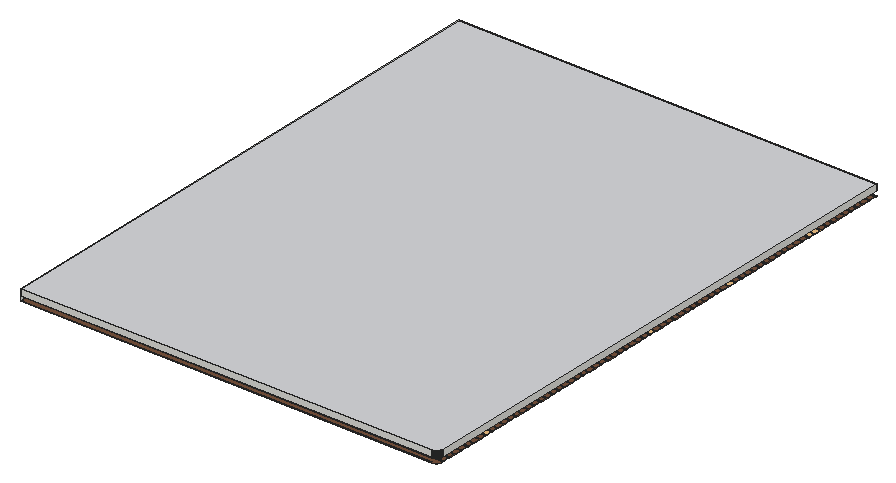
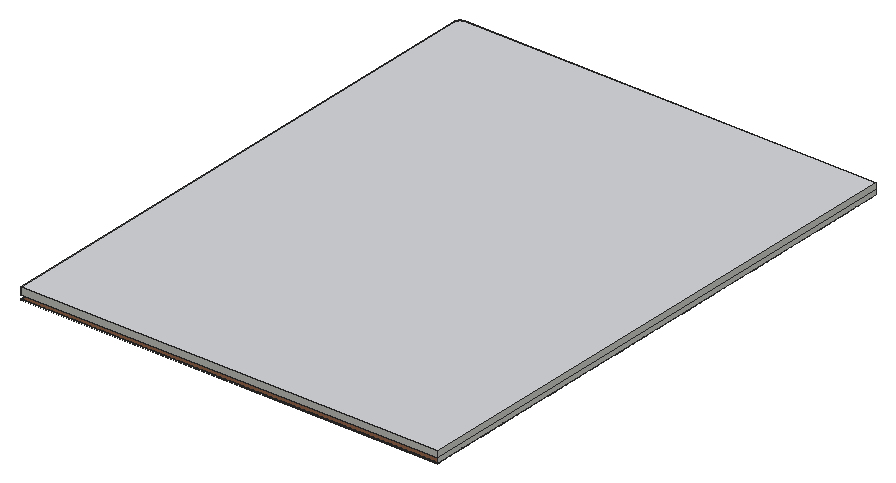
# SketchUp Ruby script. Lengths in inches.
U = 1.inch
M = Sketchup.active_model
def pt(a) = Geom::Point3d.new(a.map { |v| v * U })
def face(e, loops, mat)
  f = e.add_face(loops[0].map { |a| pt(a) })
  loops[1..].each { |l| e.add_face(l.map { |a| pt(a) }).erase! }
  f.material = f.back_material = mat if mat
  f
end
# faces: each face lists its corners as indices into pts; further lists are holes
def faces(e, pts, list, mat = nil) = list.each { |f| face(e, (f[0].is_a?(Array) ? f : [f]).map { |l| l.map { |i| pts[i] } }, mat) }
# xy, xz, yz: faces in a plane at the given z, y or x. An outline is a flat list of corners, or four numbers for a rectangle; further outlines are holes
def ring(l) = l.size == 4 ? [[l[0], l[1]], [l[2], l[1]], [l[2], l[3]], [l[0], l[3]]] : l.each_slice(2).to_a
def flat(e, list, mat, &to3) = list.each { |f| face(e, (f[0].is_a?(Array) ? f : [f]).map { |l| ring(l).map { |u, v| to3.(u, v) } }, mat) }
def xy(e, z, list, mat = nil) = flat(e, list, mat) { |x, y| [x, y, z] }
def xz(e, y, list, mat = nil) = flat(e, list, mat) { |x, z| [x, y, z] }
def yz(e, x, list, mat = nil) = flat(e, list, mat) { |y, z| [x, y, z] }
def lines(e, pts, list) = list.each { |a, b| e.add_line(pt(pts[a]), pt(pts[b])) }
# prism: a flat outline (further loops are holes) pulled along v
def prism(e, loops, v, mat = nil)
  f = face(e, loops, mat); d = Geom::Vector3d.new(v.map { |x| x * U })
  f.pushpull(f.normal.samedirection?(d) ? d.length : -d.length)
end
def box(e, o, s, mat = nil) = prism(e, [[o, [o[0] + s[0], o[1], o[2]], [o[0] + s[0], o[1] + s[1], o[2]], [o[0], o[1] + s[1], o[2]]]], [0, 0, s[2]], mat)
def at(x, y, z, deg = 0) = Geom::Transformation.translation(pt([x, y, z])) * Geom::Transformation.rotation(ORIGIN, Z_AXIS, deg.degrees)
def axes(o, x, y, z) = Geom::Transformation.new([*x, 0, *y, 0, *z, 0, *pt(o).to_a, 1])
def part(name) = M.definitions.add(name)
# library, detail: a bought-in or finely detailed component or shape, given as its bounding box
def library(name, o, s) = part(name).tap { |d| box(d.entities, o, s) }
def detail(e, o, s) = box(e.add_group.entities, o, s)
def put(e, d, t, mat = nil) = e.add_instance(d, t).tap { |i| i.material = mat if mat }
def group(e, t, mat = nil) = e.add_group.tap { |g| g.transformation = t; g.material = mat if mat }.entities
root = M.entities
M.materials.add("[Marble Carrara Floor Tile]").color = [214, 215, 218]
M.materials.add("[Wood Veneer 02]").color = [118, 81, 59]
c1 = part("Group396\#1")
xy(c1.entities,0,[[-192,-252,-192,-246,192,-246,192,-246.22,191.95,-246.77,191.93,-246.88,191.92,-246.99,191.9,-247.1,191.85,-247.32,191.83,-247.43,191.8,-247.54,191.77,-247.64,191.74,-247.75,191.71,-247.85,191.67,-247.96,191.63,-248.0625,191.59,-248.17,191.47,-248.47,191.27,-248.87,191.21,-248.97,191.16,-249.0625,191.1,-249.16,190.98,-249.34,190.92,-249.4375,190.85,-249.53,190.79,-249.62,190.72,-249.7,190.65,-249.79,190.51,-249.96,190.43,-250.04,190.36,-250.125,190.28,-250.2,190.2,-250.28,190.125,-250.36,190.04,-250.43,189.96,-250.51,189.79,-250.65,189.7,-250.72,189.62,-250.79,189.53,-250.85,189.4375,-250.92,189.34,-250.98,189.16,-251.1,189.0625,-251.16,188.97,-251.21,188.87,-251.27,188.47,-251.47,188.17,-251.59,188.0625,-251.63,187.96,-251.67,187.85,-251.71,187.75,-251.74,187.64,-251.77,187.54,-251.8,187.43,-251.83,187.32,-251.85,187.1,-251.9,186.99,-251.92,186.88,-251.93,186.77,-251.95,186.22,-252]])
xy(c1.entities,0.25,[[-192,-252,186.22,-252,186.77,-251.95,186.88,-251.93,186.99,-251.92,187.1,-251.9,187.32,-251.85,187.43,-251.83,187.54,-251.8,187.64,-251.77,187.75,-251.74,187.85,-251.71,187.96,-251.67,188.0625,-251.63,188.17,-251.59,188.47,-251.47,188.87,-251.27,188.97,-251.21,189.0625,-251.16,189.16,-251.1,189.34,-250.98,189.4375,-250.92,189.53,-250.85,189.62,-250.79,189.7,-250.72,189.79,-250.65,189.96,-250.51,190.04,-250.43,190.125,-250.36,190.2,-250.28,190.28,-250.2,190.36,-250.125,190.43,-250.04,190.51,-249.96,190.65,-249.79,190.72,-249.7,190.79,-249.62,190.85,-249.53,190.92,-249.4375,190.98,-249.34,191.1,-249.16,191.16,-249.0625,191.21,-248.97,191.27,-248.87,191.47,-248.47,191.59,-248.17,191.63,-248.0625,191.67,-247.96,191.71,-247.85,191.74,-247.75,191.77,-247.64,191.8,-247.54,191.83,-247.43,191.85,-247.32,191.9,-247.1,191.92,-246.99,191.93,-246.88,191.95,-246.77,192,-246.22,192,-246,-192,-246]])
xz(c1.entities,-252,[[-192,0,186,0.25]])
xz(c1.entities,-246,[[-192,0,192,0.25]])
yz(c1.entities,-192,[[-252,0,-246,0.25]])
c2 = part("Group397\#1")
box(c2.entities,[-192,-245,0],[384,6,0.25])
c3 = part("Group398\#1")
box(c3.entities,[-192,-238,0],[384,6,0.25])
c4 = part("Group399\#1")
box(c4.entities,[-192,-231,0],[384,6,0.25])
c5 = part("Group400\#1")
box(c5.entities,[-192,-224,0],[384,6,0.25])
c6 = part("Group401\#1")
box(c6.entities,[-192,-217,0],[384,6,0.25])
c7 = part("Group402\#1")
box(c7.entities,[-192,-210,0],[384,6,0.25])
c8 = part("Group403\#1")
box(c8.entities,[-192,-203,0],[384,6,0.25])
c9 = library("Group404\#1",[-192,-196,0],[384,6.01,0.25])
c10 = part("Group405\#1")
box(c10.entities,[-192,-189,0],[384,6,0.25])
c11 = part("Group406\#1")
box(c11.entities,[-192,-182,0],[384,6,0.25])
c12 = part("Group407\#1")
box(c12.entities,[-192,-175,0],[384,6,0.25])
c13 = part("Group408\#1")
box(c13.entities,[-192,-168,0],[384,6,0.25])
c14 = part("Group409\#1")
box(c14.entities,[-192,-161,0],[384,6,0.25])
c15 = part("Group410\#1")
box(c15.entities,[-192,-154,0],[384,6,0.25])
c16 = part("Group411\#1")
box(c16.entities,[-192,-147,0],[384,6,0.25])
c17 = part("Group412\#1")
box(c17.entities,[-192,-140,0],[384,6,0.25])
c18 = part("Group413\#1")
box(c18.entities,[-192,-133,0],[384,6,0.25])
c19 = part("Group414\#1")
box(c19.entities,[-192,-126,0],[384,6,0.25])
c20 = part("Group415\#1")
box(c20.entities,[-192,-119,0],[384,6,0.25])
c21 = part("Group416\#1")
box(c21.entities,[-192,-112,0],[384,6,0.25])
c22 = part("Group417\#1")
box(c22.entities,[-192,-105,0],[384,6,0.25])
c23 = part("Group418\#1")
box(c23.entities,[-192,-98,0],[384,6,0.25])
c24 = part("Group419\#1")
box(c24.entities,[-192,-91,0],[384,6,0.25])
c25 = part("Group420\#1")
box(c25.entities,[-192,-84,0],[384,6,0.25])
c26 = part("Group421\#1")
box(c26.entities,[-192,-77,0],[384,6,0.25])
c27 = part("Group422\#1")
box(c27.entities,[-192,-70,0],[384,6,0.25])
c28 = part("Group423\#1")
box(c28.entities,[-192,-63,0],[384,6,0.25])
c29 = part("Group424\#1")
box(c29.entities,[-192,-56,0],[384,6,0.25])
c30 = part("Group425\#1")
box(c30.entities,[-192,-49,0],[384,6,0.25])
c31 = part("Group426\#1")
box(c31.entities,[-192,-42,0],[384,6,0.25])
c32 = part("Group427\#1")
box(c32.entities,[-192,-35,0],[384,6,0.25])
c33 = part("Group428\#1")
box(c33.entities,[-192,-28,0],[384,6,0.25])
c34 = part("Group429\#1")
box(c34.entities,[-192,-21,0],[384,6,0.25])
c35 = part("Group430\#1")
box(c35.entities,[-192,-14,0],[384,6,0.25])
c36 = library("Group431\#1",[-192,-7,0],[384,6,0.25])
c37 = part("Group432\#1")
box(c37.entities,[-192,0,0],[384,6,0.25])
c38 = part("Group433\#1")
box(c38.entities,[-192,7,0],[384,6,0.25])
c39 = part("Group434\#1")
box(c39.entities,[-192,14,0],[384,6,0.25])
c40 = part("Group435\#1")
box(c40.entities,[-192,21,0],[384,6,0.25])
c41 = part("Group436\#1")
box(c41.entities,[-192,28,0],[384,6,0.25])
c42 = part("Group437\#1")
box(c42.entities,[-192,35,0],[384,6,0.25])
c43 = part("Group438\#1")
box(c43.entities,[-192,42,0],[384,6,0.25])
c44 = part("Group439\#1")
box(c44.entities,[-192,49,0],[384,6,0.25])
c45 = part("Group440\#1")
box(c45.entities,[-192,56,0],[384,6,0.25])
c46 = part("Group441\#1")
box(c46.entities,[-192,63,0],[384,6,0.25])
c47 = part("Group442\#1")
box(c47.entities,[-192,70,0],[384,6,0.25])
c48 = part("Group443\#1")
box(c48.entities,[-192,77,0],[384,6,0.25])
c49 = library("Group444\#1",[-192,84,0],[384,6,0.25])
c50 = part("Group445\#1")
box(c50.entities,[-192,91,0],[384,6,0.25])
c51 = part("Group446\#1")
box(c51.entities,[-192,98,0],[384,6,0.25])
c52 = part("Group447\#1")
box(c52.entities,[-192,105,0],[384,6,0.25])
c53 = part("Group448\#1")
box(c53.entities,[-192,112,0],[384,6,0.25])
c54 = part("Group449\#1")
box(c54.entities,[-192,119,0],[384,6,0.25])
c55 = part("Group450\#1")
box(c55.entities,[-192,126,0],[384,6,0.25])
c56 = part("Group451\#1")
box(c56.entities,[-192,133,0],[384,6,0.25])
c57 = part("Group452\#1")
box(c57.entities,[-192,140,0],[384,6,0.25])
c58 = part("Group453\#1")
box(c58.entities,[-192,147,0],[384,6,0.25])
c59 = part("Group454\#1")
box(c59.entities,[-192,154,0],[384,6,0.25])
c60 = part("Group455\#1")
box(c60.entities,[-192,161,0],[384,6,0.25])
c61 = part("Group456\#1")
box(c61.entities,[-192,168,0],[384,6,0.25])
c62 = library("Group458\#1",[-192,182,0],[384,6,0.25])
c63 = part("Group459\#1")
box(c63.entities,[-192,189,0],[384,6,0.25])
c64 = part("Group460\#1")
box(c64.entities,[-192,196,0],[384,6,0.25])
c65 = part("Group461\#1")
box(c65.entities,[-192,203,0],[384,6,0.25])
c66 = part("Group462\#1")
box(c66.entities,[-192,210,0],[384,6,0.25])
c67 = part("Group463\#1")
box(c67.entities,[-192,217,0],[384,6,0.25])
c68 = part("Group464\#1")
box(c68.entities,[-192,224,0],[384,6,0.25])
c69 = part("Group465\#1")
box(c69.entities,[-192,231,0],[384,6,0.25])
c70 = part("Group466\#1")
box(c70.entities,[-192,238,0],[384,6,0.25])
c71 = part("Group467\#1")
box(c71.entities,[-192,245,0],[384,6,0.25])
c72 = part("Group468\#1")
xz(c72.entities,252,[[-192,0,192,0.25]])
c73 = library("Group457\#1",[-192,175,0],[384,6,0.25])
c74 = part("Group394\#1")
put(c74.entities,c1,at(0,0,0))
put(c74.entities,c2,at(0,0,0))
put(c74.entities,c3,at(0,0,0))
put(c74.entities,c4,at(0,0,0))
put(c74.entities,c5,at(0,0,0))
put(c74.entities,c6,at(0,0,0))
put(c74.entities,c7,at(0,0,0))
put(c74.entities,c8,at(0,0,0))
put(c74.entities,c9,at(0,0,0))
put(c74.entities,c10,at(0,0,0))
put(c74.entities,c11,at(0,0,0))
put(c74.entities,c12,at(0,0,0))
put(c74.entities,c13,at(0,0,0))
put(c74.entities,c14,at(0,0,0))
put(c74.entities,c15,at(0,0,0))
put(c74.entities,c16,at(0,0,0))
put(c74.entities,c17,at(0,0,0))
put(c74.entities,c18,at(0,0,0))
put(c74.entities,c19,at(0,0,0))
put(c74.entities,c20,at(0,0,0))
put(c74.entities,c21,at(0,0,0))
put(c74.entities,c22,at(0,0,0))
put(c74.entities,c23,at(0,0,0))
put(c74.entities,c24,at(0,0,0))
put(c74.entities,c25,at(0,0,0))
put(c74.entities,c26,at(0,0,0))
put(c74.entities,c27,at(0,0,0))
put(c74.entities,c28,at(0,0,0))
put(c74.entities,c29,at(0,0,0))
put(c74.entities,c30,at(0,0,0))
put(c74.entities,c31,at(0,0,0))
put(c74.entities,c32,at(0,0,0))
put(c74.entities,c33,at(0,0,0))
put(c74.entities,c34,at(0,0,0))
put(c74.entities,c35,at(0,0,0))
put(c74.entities,c36,at(0,0,0))
put(c74.entities,c37,at(0,0,0))
put(c74.entities,c38,at(0,0,0))
put(c74.entities,c39,at(0,0,0))
put(c74.entities,c40,at(0,0,0))
put(c74.entities,c41,at(0,0,0))
put(c74.entities,c42,at(0,0,0))
put(c74.entities,c43,at(0,0,0))
put(c74.entities,c44,at(0,0,0))
put(c74.entities,c45,at(0,0,0))
put(c74.entities,c46,at(0,0,0))
put(c74.entities,c47,at(0,0,0))
put(c74.entities,c48,at(0,0,0))
put(c74.entities,c49,at(0,0,0))
put(c74.entities,c50,at(0,0,0))
put(c74.entities,c51,at(0,0,0))
put(c74.entities,c52,at(0,0,0))
put(c74.entities,c53,at(0,0,0))
put(c74.entities,c54,at(0,0,0))
put(c74.entities,c55,at(0,0,0))
put(c74.entities,c56,at(0,0,0))
put(c74.entities,c57,at(0,0,0))
put(c74.entities,c58,at(0,0,0))
put(c74.entities,c59,at(0,0,0))
put(c74.entities,c60,at(0,0,0))
put(c74.entities,c61,at(0,0,0))
put(c74.entities,c62,at(0,0,0))
put(c74.entities,c63,at(0,0,0))
put(c74.entities,c64,at(0,0,0))
put(c74.entities,c65,at(0,0,0))
put(c74.entities,c66,at(0,0,0))
put(c74.entities,c67,at(0,0,0))
put(c74.entities,c68,at(0,0,0))
put(c74.entities,c69,at(0,0,0))
put(c74.entities,c70,at(0,0,0))
put(c74.entities,c71,at(0,0,0))
put(c74.entities,c72,at(0,0,0))
put(c74.entities,c73,at(0,0,0))
xz(root,525,[[279.84,128,279.92,129],[279.92,128,280,129],[280,128,280.08,129],[280.08,128,280.16,129]])
yz(root,48,[[96,128,600,132]])
yz(root,357,[[341.84,128,341.92,129],[341.92,128,342,129],[342,128,342.08,129],[342.08,128,342.16,129],[434.84,128,434.92,129],
  [434.92,128,435,129],[435,128,435.08,129],[435.08,128,435.16,129]])
p = [[357.05,249.55,128],[357.07,249.625,128],[357.07,249.625,129],[357.05,249.55,129],[357.08,249.7,128],[357.08,249.7,129],
  [357.1,249.78,128],[357.1,249.78,129],[357.125,249.85,128],[357.125,249.85,129],[357.15,249.93,128],[357.15,249.93,129],
  [357.17,250,128],[357.17,250,129],[357.2,250.08,128],[357.2,250.08,129],[357.23,250.15,128],[357.23,250.15,129],
  [357.26,250.22,128],[357.26,250.22,129],[357.29,250.29,128],[357.29,250.29,129],[357.33,250.36,128],[357.33,250.36,129],
  [357.36,250.43,128],[357.36,250.43,129],[357.4,250.5,128],[357.4,250.5,129],[357.44,250.57,128],[357.44,250.57,129],
  [357.48,250.63,128],[357.48,250.63,129],[357.53,250.7,128],[357.53,250.7,129],[357.57,250.76,128],[357.57,250.76,129],
  [357.57,340.24,128],[357.53,340.3,128],[357.53,340.3,129],[357.57,340.24,129],[357.48,340.37,128],[357.48,340.37,129],
  [357.44,340.43,128],[357.4,340.5,128],[357.4,340.5,129],[357.44,340.43,129],[357.36,340.57,128],[357.36,340.57,129],
  [357.33,340.64,128],[357.29,340.71,128],[357.29,340.71,129],[357.33,340.64,129],[357.26,340.78,128],[357.26,340.78,129],
  [357.23,340.85,128],[357.23,340.85,129],[357.2,340.92,128],[357.17,341,128],[357.17,341,129],[357.2,340.92,129],
  [357.15,341.07,128],[357.15,341.07,129],[357.125,341.15,128],[357.1,341.22,128],[357.1,341.22,129],[357.125,341.15,129],
  [357.08,341.3,128],[357.08,341.3,129],[357.07,341.375,128],[357.07,341.375,129],[357.05,341.45,128],[357.05,341.45,129],
  [357.04,341.53,128],[357.03,341.61,128],[357.03,341.61,129],[357.04,341.53,129],[357.02,341.6875,128],[357.02,341.6875,129],
  [357.01,341.76,128],[357.01,341.76,129],[357,341.84,128],[357,341.84,129],[357,342.16,128],[357.01,342.24,128],
  [357.01,342.24,129],[357,342.16,129],[357.02,342.3125,128],[357.02,342.3125,129],[357.03,342.39,128],[357.03,342.39,129],
  [357.04,342.47,128],[357.04,342.47,129],[357.05,342.55,128],[357.05,342.55,129],[357.07,342.625,128],[357.07,342.625,129],
  [357.08,342.7,128],[357.08,342.7,129],[357.1,342.78,128],[357.1,342.78,129],[357.125,342.85,128],[357.125,342.85,129],
  [357.15,342.93,128],[357.15,342.93,129],[357.17,343,128],[357.17,343,129],[357.2,343.08,128],[357.2,343.08,129],
  [357.23,343.15,128],[357.23,343.15,129],[357.26,343.22,128],[357.26,343.22,129],[357.29,343.29,128],[357.29,343.29,129],
  [357.33,343.36,128],[357.33,343.36,129],[357.36,343.43,128],[357.36,343.43,129],[357.4,343.5,128],[357.4,343.5,129],
  [357.44,343.57,128],[357.44,343.57,129],[357.48,343.63,128],[357.48,343.63,129],[357.53,343.7,128],[357.53,343.7,129],
  [357.53,433.3,128],[357.48,433.37,128],[357.48,433.37,129],[357.53,433.3,129],[357.44,433.43,128],[357.4,433.5,128],
  [357.4,433.5,129],[357.44,433.43,129],[357.36,433.57,128],[357.36,433.57,129],[357.33,433.64,128],[357.29,433.71,128],
  [357.29,433.71,129],[357.33,433.64,129],[357.26,433.78,128],[357.26,433.78,129],[357.23,433.85,128],[357.23,433.85,129],
  [357.2,433.92,128],[357.17,434,128],[357.17,434,129],[357.2,433.92,129],[357.15,434.07,128],[357.15,434.07,129],
  [357.125,434.15,128],[357.1,434.22,128],[357.1,434.22,129],[357.125,434.15,129],[357.08,434.3,128],[357.08,434.3,129],
  [357.07,434.375,128],[357.07,434.375,129],[357.05,434.45,128],[357.05,434.45,129],[357.04,434.53,128],[357.03,434.61,128],
  [357.03,434.61,129],[357.04,434.53,129],[357.02,434.6875,128],[357.02,434.6875,129],[357.01,434.76,128],[357.01,434.76,129],
  [357,434.84,128],[357,434.84,129],[357,435.16,128],[357.01,435.24,128],[357.01,435.24,129],[357,435.16,129],
  [357.02,435.3125,128],[357.02,435.3125,129],[357.03,435.39,128],[357.03,435.39,129],[357.04,435.47,128],[357.04,435.47,129],
  [357.05,435.55,128],[357.05,435.55,129],[357.07,435.625,128],[357.07,435.625,129],[357.08,435.7,128],[357.08,435.7,129],
  [357.1,435.78,128],[357.1,435.78,129],[357.125,435.85,128],[357.125,435.85,129],[357.15,435.93,128],[357.15,435.93,129],
  [357.17,436,128],[357.17,436,129],[357.2,436.08,128],[357.2,436.08,129],[357.23,436.15,128],[357.23,436.15,129],
  [357.26,436.22,128],[357.26,436.22,129],[357.29,436.29,128],[357.29,436.29,129],[357.33,436.36,128],[357.33,436.36,129],
  [357.36,436.43,128],[357.36,436.43,129],[357.4,436.5,128],[357.4,436.5,129],[357.44,436.57,128],[357.44,436.57,129],
  [357.48,436.63,128],[357.48,436.63,129],[357.53,436.7,128],[357.53,436.7,129],[279.53,525.04,128],[279.45,525.05,128],
  [279.45,525.05,129],[279.53,525.04,129],[279.61,525.03,128],[279.61,525.03,129],[279.6875,525.02,128],[279.6875,525.02,129],
  [279.76,525.01,128],[279.76,525.01,129],[279.84,525,128],[279.84,525,129],[280.24,525.01,128],[280.16,525,128],
  [280.16,525,129],[280.24,525.01,129],[280.3125,525.02,128],[280.3125,525.02,129],[280.39,525.03,128],[280.39,525.03,129],
  [280.47,525.04,128],[280.47,525.04,129],[280.55,525.05,128],[280.55,525.05,129],[279.07,525.15,128],[279,525.17,128],
  [279,525.17,129],[279.07,525.15,129],[279.15,525.125,128],[279.15,525.125,129],[279.22,525.1,128],[279.22,525.1,129],
  [279.3,525.08,128],[279.3,525.08,129],[279.375,525.07,128],[279.375,525.07,129],[280.625,525.07,128],[280.625,525.07,129],
  [280.7,525.08,128],[280.7,525.08,129],[280.78,525.1,128],[280.78,525.1,129],[280.85,525.125,128],[280.85,525.125,129],
  [280.93,525.15,128],[280.93,525.15,129],[281,525.17,128],[281,525.17,129],[278.85,525.23,128],[278.78,525.26,128],
  [278.78,525.26,129],[278.85,525.23,129],[278.92,525.2,128],[278.92,525.2,129],[281.08,525.2,128],[281.08,525.2,129],
  [281.15,525.23,128],[281.15,525.23,129],[281.22,525.26,128],[281.22,525.26,129],[278.71,525.29,128],[278.64,525.33,128],
  [278.64,525.33,129],[278.71,525.29,129],[281.29,525.29,128],[281.29,525.29,129],[281.36,525.33,128],[281.36,525.33,129]]
faces(root,p,[[0,1,2,3],[1,4,5,2],[4,6,7,5],[6,8,9,7],[8,10,11,9],[10,12,13,11],[12,14,15,13],[14,16,17,15],
  [16,18,19,17],[18,20,21,19],[20,22,23,21],[22,24,25,23],[24,26,27,25],[26,28,29,27],[28,30,31,29],[30,32,33,31],
  [32,34,35,33],[36,37,38,39],[37,40,41,38],[42,43,44,45],[40,42,45,41],[43,46,47,44],[48,49,50,51],[46,48,51,47],
  [49,52,53,50],[52,54,55,53],[56,57,58,59],[54,56,59,55],[57,60,61,58],[62,63,64,65],[60,62,65,61],[63,66,67,64],
  [66,68,69,67],[68,70,71,69],[72,73,74,75],[70,72,75,71],[73,76,77,74],[76,78,79,77],[78,80,81,79],[82,83,84,85],
  [83,86,87,84],[86,88,89,87],[88,90,91,89],[90,92,93,91],[92,94,95,93],[94,96,97,95],[96,98,99,97],[98,100,101,99],
  [100,102,103,101],[102,104,105,103],[104,106,107,105],[106,108,109,107],[108,110,111,109],[110,112,113,111],[112,114,115,113],[114,116,117,115],
  [116,118,119,117],[118,120,121,119],[120,122,123,121],[122,124,125,123],[126,127,128,129],[130,131,132,133],[127,130,133,128],[131,134,135,132],
  [136,137,138,139],[134,136,139,135],[137,140,141,138],[140,142,143,141],[144,145,146,147],[142,144,147,143],[145,148,149,146],[150,151,152,153],
  [148,150,153,149],[151,154,155,152],[154,156,157,155],[156,158,159,157],[160,161,162,163],[158,160,163,159],[161,164,165,162],[164,166,167,165],
  [166,168,169,167],[170,171,172,173],[171,174,175,172],[174,176,177,175],[176,178,179,177],[178,180,181,179],[180,182,183,181],[182,184,185,183],
  [184,186,187,185],[186,188,189,187],[188,190,191,189],[190,192,193,191],[192,194,195,193],[194,196,197,195],[196,198,199,197],[198,200,201,199],
  [200,202,203,201],[202,204,205,203],[204,206,207,205],[206,208,209,207],[208,210,211,209],[210,212,213,211],[214,215,216,217],[218,214,217,219],
  [220,218,219,221],[222,220,221,223],[224,222,223,225],[226,227,228,229],[230,226,229,231],[232,230,231,233],[234,232,233,235],[236,234,235,237],
  [238,239,240,241],[242,238,241,243],[244,242,243,245],[246,244,245,247],[248,246,247,249],[215,248,249,216],[250,236,237,251],[252,250,251,253],
  [254,252,253,255],[256,254,255,257],[258,256,257,259],[260,258,259,261],[262,263,264,265],[266,262,265,267],[239,266,267,240],[268,260,261,269],
  [270,268,269,271],[272,270,271,273],[274,275,276,277],[263,274,277,264],[278,272,273,279],[280,278,279,281]])
put(root,c74,at(240,348,127.75),"[Wood Veneer 02]")
g1 = group(root,at(57,105,138))
xy(g1,-6,[[-9,-9,-9,495,375,495,375,-3.22,374.95,-3.77,374.93,-3.88,374.92,-3.99,374.9,-4.1,374.85,-4.32,374.83,-4.43,374.8,-4.54,374.77,-4.64,374.74,-4.75,374.71,-4.85,374.67,-4.96,374.63,-5.0625,374.59,-5.17,374.47,-5.47,374.27,-5.87,374.21,-5.97,374.16,-6.0625,374.1,-6.16,373.98,-6.34,373.92,-6.4375,373.85,-6.53,373.79,-6.62,373.72,-6.7,373.65,-6.79,373.51,-6.96,373.43,-7.04,373.36,-7.125,373.28,-7.2,373.2,-7.28,373.125,-7.36,373.04,-7.43,372.96,-7.51,372.79,-7.65,372.7,-7.72,372.62,-7.79,372.53,-7.85,372.4375,-7.92,372.34,-7.98,372.16,-8.1,372.0625,-8.16,371.97,-8.21,371.87,-8.27,371.47,-8.47,371.17,-8.59,371.0625,-8.63,370.96,-8.67,370.85,-8.71,370.75,-8.74,370.64,-8.77,370.54,-8.8,370.43,-8.83,370.32,-8.85,370.1,-8.9,369.99,-8.92,369.88,-8.93,369.77,-8.95,369.22,-9]])
xy(g1,0,[[-9,-9,369.22,-9,369.77,-8.95,369.88,-8.93,369.99,-8.92,370.1,-8.9,370.32,-8.85,370.43,-8.83,370.54,-8.8,370.64,-8.77,370.75,-8.74,370.85,-8.71,370.96,-8.67,371.0625,-8.63,371.17,-8.59,371.47,-8.47,371.87,-8.27,371.97,-8.21,372.0625,-8.16,372.16,-8.1,372.34,-7.98,372.4375,-7.92,372.53,-7.85,372.62,-7.79,372.7,-7.72,372.79,-7.65,372.96,-7.51,373.04,-7.43,373.125,-7.36,373.2,-7.28,373.28,-7.2,373.36,-7.125,373.43,-7.04,373.51,-6.96,373.65,-6.79,373.72,-6.7,373.79,-6.62,373.85,-6.53,373.92,-6.4375,373.98,-6.34,374.1,-6.16,374.16,-6.0625,374.21,-5.97,374.27,-5.87,374.47,-5.47,374.59,-5.17,374.63,-5.0625,374.67,-4.96,374.71,-4.85,374.74,-4.75,374.77,-4.64,374.8,-4.54,374.83,-4.43,374.85,-4.32,374.9,-4.1,374.92,-3.99,374.93,-3.88,374.95,-3.77,375,-3.22,375,495,-9,495]],"[Marble Carrara Floor Tile]")
xz(g1,-9,[[-9,-6,369,0],[369,-6,369.11,0],[369.11,-6,369.22,0]])
xz(g1,495,[[-9,-6,375,0]])
yz(g1,-9,[[-9,-6,495,0]])
yz(g1,375,[[-3.22,-6,-3.11,0],[-3.11,-6,-3,0],[-3,-6,495,0]])
p = [[369.33,-8.99,0],[369.22,-9,0],[369.22,-9,-6],[369.33,-8.99,-6],[369.44,-8.98,0],[369.44,-8.98,-6],
  [369.55,-8.97,0],[369.55,-8.97,-6],[369.66,-8.96,0],[369.66,-8.96,-6],[369.77,-8.95,0],[369.77,-8.95,-6],
  [369.88,-8.93,0],[369.88,-8.93,-6],[369.99,-8.92,0],[369.99,-8.92,-6],[370.1,-8.9,0],[370.1,-8.9,-6],
  [370.21,-8.875,0],[370.21,-8.875,-6],[370.32,-8.85,0],[370.32,-8.85,-6],[370.43,-8.83,0],[370.43,-8.83,-6],
  [370.54,-8.8,0],[370.54,-8.8,-6],[370.64,-8.77,0],[370.64,-8.77,-6],[370.75,-8.74,0],[370.75,-8.74,-6],
  [370.85,-8.71,0],[370.85,-8.71,-6],[370.96,-8.67,0],[370.96,-8.67,-6],[371.0625,-8.63,0],[371.0625,-8.63,-6],
  [371.17,-8.59,0],[371.17,-8.59,-6],[371.27,-8.55,0],[371.27,-8.55,-6],[371.37,-8.51,0],[371.37,-8.51,-6],
  [371.47,-8.47,0],[371.47,-8.47,-6],[371.57,-8.42,0],[371.57,-8.42,-6],[371.67,-8.37,0],[371.67,-8.37,-6],
  [371.77,-8.32,0],[371.77,-8.32,-6],[371.87,-8.27,0],[371.87,-8.27,-6],[371.97,-8.21,0],[371.97,-8.21,-6],
  [372.0625,-8.16,0],[372.0625,-8.16,-6],[372.16,-8.1,0],[372.16,-8.1,-6],[372.25,-8.04,0],[372.25,-8.04,-6],
  [372.4375,-7.92,0],[372.34,-7.98,0],[372.34,-7.98,-6],[372.4375,-7.92,-6],[372.53,-7.85,0],[372.53,-7.85,-6],
  [372.62,-7.79,0],[372.62,-7.79,-6],[372.7,-7.72,0],[372.7,-7.72,-6],[372.79,-7.65,0],[372.79,-7.65,-6],
  [372.875,-7.58,0],[372.875,-7.58,-6],[372.96,-7.51,0],[372.96,-7.51,-6],[373.04,-7.43,0],[373.04,-7.43,-6],
  [373.125,-7.36,0],[373.125,-7.36,-6],[373.2,-7.28,0],[373.2,-7.28,-6],[373.28,-7.2,0],[373.28,-7.2,-6],
  [373.36,-7.125,0],[373.36,-7.125,-6],[373.43,-7.04,0],[373.43,-7.04,-6],[373.51,-6.96,0],[373.51,-6.96,-6],
  [373.58,-6.875,0],[373.58,-6.875,-6],[373.65,-6.79,0],[373.65,-6.79,-6],[373.72,-6.7,0],[373.72,-6.7,-6],
  [373.79,-6.62,0],[373.79,-6.62,-6],[373.85,-6.53,0],[373.85,-6.53,-6],[373.92,-6.4375,0],[373.92,-6.4375,-6],
  [373.98,-6.34,0],[373.98,-6.34,-6],[374.1,-6.16,0],[374.04,-6.25,0],[374.04,-6.25,-6],[374.1,-6.16,-6],
  [374.16,-6.0625,0],[374.16,-6.0625,-6],[374.21,-5.97,0],[374.21,-5.97,-6],[374.27,-5.87,0],[374.27,-5.87,-6],
  [374.32,-5.77,0],[374.32,-5.77,-6],[374.37,-5.67,0],[374.37,-5.67,-6],[374.42,-5.57,0],[374.42,-5.57,-6],
  [374.47,-5.47,0],[374.47,-5.47,-6],[374.51,-5.37,0],[374.51,-5.37,-6],[374.55,-5.27,0],[374.55,-5.27,-6],
  [374.59,-5.17,0],[374.59,-5.17,-6],[374.63,-5.0625,0],[374.63,-5.0625,-6],[374.67,-4.96,0],[374.67,-4.96,-6],
  [374.71,-4.85,0],[374.71,-4.85,-6],[374.74,-4.75,0],[374.74,-4.75,-6],[374.77,-4.64,0],[374.77,-4.64,-6],
  [374.8,-4.54,0],[374.8,-4.54,-6],[374.83,-4.43,0],[374.83,-4.43,-6],[374.85,-4.32,0],[374.85,-4.32,-6],
  [374.875,-4.21,0],[374.875,-4.21,-6],[374.9,-4.1,0],[374.9,-4.1,-6],[374.92,-3.99,0],[374.92,-3.99,-6],
  [374.93,-3.88,0],[374.93,-3.88,-6],[374.95,-3.77,0],[374.95,-3.77,-6],[374.96,-3.66,0],[374.96,-3.66,-6],
  [374.97,-3.55,0],[374.97,-3.55,-6],[374.98,-3.44,0],[374.98,-3.44,-6],[374.99,-3.33,0],[374.99,-3.33,-6],
  [375,-3.22,0],[375,-3.22,-6]]
faces(g1,p,[[0,1,2,3],[4,0,3,5],[6,4,5,7],[8,6,7,9],[10,8,9,11],[12,10,11,13],[14,12,13,15],[16,14,15,17],
  [18,16,17,19],[20,18,19,21],[22,20,21,23],[24,22,23,25],[26,24,25,27],[28,26,27,29],[30,28,29,31],[32,30,31,33],
  [34,32,33,35],[36,34,35,37],[38,36,37,39],[40,38,39,41],[42,40,41,43],[44,42,43,45],[46,44,45,47],[48,46,47,49],
  [50,48,49,51],[52,50,51,53],[54,52,53,55],[56,54,55,57],[58,56,57,59],[60,61,62,63],[61,58,59,62],[64,60,63,65],
  [66,64,65,67],[68,66,67,69],[70,68,69,71],[72,70,71,73],[74,72,73,75],[76,74,75,77],[78,76,77,79],[80,78,79,81],
  [82,80,81,83],[84,82,83,85],[86,84,85,87],[88,86,87,89],[90,88,89,91],[92,90,91,93],[94,92,93,95],[96,94,95,97],
  [98,96,97,99],[100,98,99,101],[102,100,101,103],[104,105,106,107],[105,102,103,106],[108,104,107,109],[110,108,109,111],[112,110,111,113],
  [114,112,113,115],[116,114,115,117],[118,116,117,119],[120,118,119,121],[122,120,121,123],[124,122,123,125],[126,124,125,127],[128,126,127,129],
  [130,128,129,131],[132,130,131,133],[134,132,133,135],[136,134,135,137],[138,136,137,139],[140,138,139,141],[142,140,141,143],[144,142,143,145],
  [146,144,145,147],[148,146,147,149],[150,148,149,151],[152,150,151,153],[154,152,153,155],[156,154,155,157],[158,156,157,159],[160,158,159,161],
  [162,160,161,163]])
